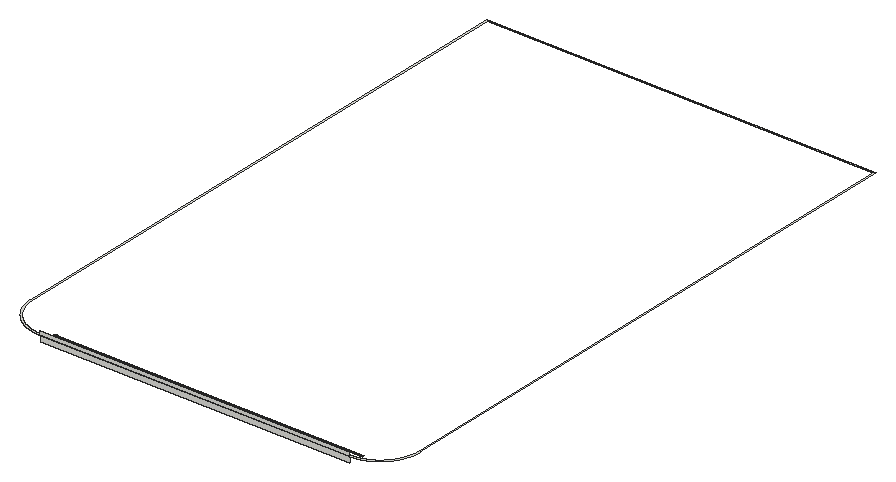
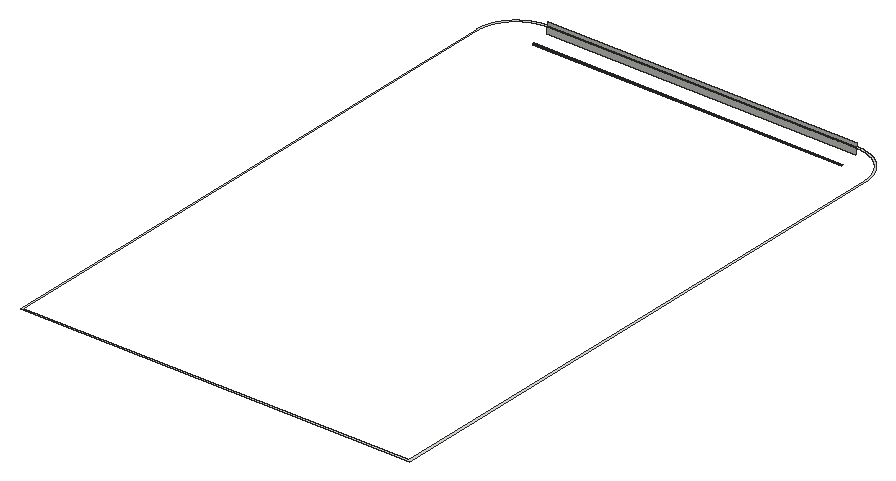
# SketchUp Ruby script. Lengths in inches.
U = 1.inch
M = Sketchup.active_model
def pt(a) = Geom::Point3d.new(a.map { |v| v * U })
def face(e, loops, mat)
  f = e.add_face(loops[0].map { |a| pt(a) })
  loops[1..].each { |l| e.add_face(l.map { |a| pt(a) }).erase! }
  f.material = f.back_material = mat if mat
  f
end
# faces: each face lists its corners as indices into pts; further lists are holes
def faces(e, pts, list, mat = nil) = list.each { |f| face(e, (f[0].is_a?(Array) ? f : [f]).map { |l| l.map { |i| pts[i] } }, mat) }
# xy, xz, yz: faces in a plane at the given z, y or x. An outline is a flat list of corners, or four numbers for a rectangle; further outlines are holes
def ring(l) = l.size == 4 ? [[l[0], l[1]], [l[2], l[1]], [l[2], l[3]], [l[0], l[3]]] : l.each_slice(2).to_a
def flat(e, list, mat, &to3) = list.each { |f| face(e, (f[0].is_a?(Array) ? f : [f]).map { |l| ring(l).map { |u, v| to3.(u, v) } }, mat) }
def xy(e, z, list, mat = nil) = flat(e, list, mat) { |x, y| [x, y, z] }
def xz(e, y, list, mat = nil) = flat(e, list, mat) { |x, z| [x, y, z] }
def yz(e, x, list, mat = nil) = flat(e, list, mat) { |y, z| [x, y, z] }
def lines(e, pts, list) = list.each { |a, b| e.add_line(pt(pts[a]), pt(pts[b])) }
# prism: a flat outline (further loops are holes) pulled along v
def prism(e, loops, v, mat = nil)
  f = face(e, loops, mat); d = Geom::Vector3d.new(v.map { |x| x * U })
  f.pushpull(f.normal.samedirection?(d) ? d.length : -d.length)
end
def box(e, o, s, mat = nil) = prism(e, [[o, [o[0] + s[0], o[1], o[2]], [o[0] + s[0], o[1] + s[1], o[2]], [o[0], o[1] + s[1], o[2]]]], [0, 0, s[2]], mat)
def at(x, y, z, deg = 0) = Geom::Transformation.translation(pt([x, y, z])) * Geom::Transformation.rotation(ORIGIN, Z_AXIS, deg.degrees)
def axes(o, x, y, z) = Geom::Transformation.new([*x, 0, *y, 0, *z, 0, *pt(o).to_a, 1])
def part(name) = M.definitions.add(name)
# library, detail: a bought-in or finely detailed component or shape, given as its bounding box
def library(name, o, s) = part(name).tap { |d| box(d.entities, o, s) }
def detail(e, o, s) = box(e.add_group.entities, o, s)
def put(e, d, t, mat = nil) = e.add_instance(d, t).tap { |i| i.material = mat if mat }
def group(e, t, mat = nil) = e.add_group.tap { |g| g.transformation = t; g.material = mat if mat }.entities
root = M.entities
xy(root,354.5,[[[38.61,204,38.21,204.01,37.82,204.02,37.43,204.04,37.04,204.0625,36.65,204.09,36.25,204.125,35.86,204.16,35.08,204.26,34.7,204.31,33.92,204.43,33.53,204.5,33.15,204.58,32.76,204.66,32.38,204.74,31.62,204.92,31.24,205.02,30.86,205.125,30.48,205.24,30.1,205.35,29.36,205.59,28.62,205.85,28.25,205.99,27.88,206.14,27.52,206.28,27.16,206.4375,26.8,206.59,26.44,206.76,26.08,206.92,25.73,207.09,25.03,207.45,24.69,207.64,24.34,207.83,24,208.02,23.66,208.22,23.33,208.42,22.99,208.63,22.66,208.84,22.33,209.06,22.01,209.28,21.6875,209.5,21.37,209.73,21.05,209.96,20.43,210.44,20.12,210.6875,19.82,210.93,19.52,211.1875,19.22,211.44,18.93,211.71,18.64,211.97,18.35,212.24,18.07,212.51,17.51,213.07,17.24,213.35,16.97,213.64,16.71,213.93,16.44,214.22,16.1875,214.52,15.93,214.82,15.6875,215.12,15.44,215.43,14.96,216.05,14.73,216.37,14.5,216.6875,14.28,217.01,14.06,217.33,13.84,217.66,13.63,217.99,13.42,218.33,13.22,218.66,13.02,219,12.83,219.34,12.64,219.69,12.45,220.03,12.09,220.73,11.92,221.08,11.76,221.44,11.59,221.8,11.4375,222.16,11.28,222.52,11.14,222.88,10.99,223.25,10.85,223.62,10.59,224.36,10.35,225.1,10.24,225.48,10.125,225.86,10.02,226.24,9.92,226.62,9.74,227.38,9.66,227.76,9.58,228.15,9.5,228.53,9.43,228.92,9.31,229.7,9.26,230.08,9.16,230.86,9.125,231.25,9.09,231.65,9.0625,232.04,9.04,232.43,9.02,232.82,9.01,233.21,9,233.61,9,660,300,660,300,233.61,299.99,233.21,299.98,232.82,299.96,232.43,299.9375,232.04,299.91,231.65,299.875,231.25,299.84,230.86,299.74,230.08,299.69,229.7,299.57,228.92,299.5,228.53,299.42,228.15,299.34,227.76,299.26,227.38,299.08,226.62,298.98,226.24,298.875,225.86,298.76,225.48,298.65,225.1,298.41,224.36,298.15,223.62,298.01,223.25,297.86,222.88,297.72,222.52,297.5625,222.16,297.41,221.8,297.24,221.44,297.08,221.08,296.91,220.73,296.55,220.03,296.36,219.69,296.17,219.34,295.98,219,295.78,218.66,295.58,218.33,295.37,217.99,295.16,217.66,294.94,217.33,294.72,217.01,294.5,216.6875,294.27,216.37,294.04,216.05,293.56,215.43,293.3125,215.12,293.07,214.82,292.8125,214.52,292.56,214.22,292.29,213.93,292.03,213.64,291.76,213.35,291.49,213.07,290.93,212.51,290.65,212.24,290.36,211.97,290.07,211.71,289.78,211.44,289.48,211.1875,289.18,210.93,288.88,210.6875,288.57,210.44,287.95,209.96,287.63,209.73,287.3125,209.5,286.99,209.28,286.67,209.06,286.34,208.84,286.01,208.63,285.67,208.42,285.34,208.22,285,208.02,284.66,207.83,284.31,207.64,283.97,207.45,283.27,207.09,282.92,206.92,282.56,206.76,282.2,206.59,281.84,206.4375,281.48,206.28,281.12,206.14,280.75,205.99,280.38,205.85,279.64,205.59,278.9,205.35,278.52,205.24,278.14,205.125,277.76,205.02,277.38,204.92,276.62,204.74,276.24,204.66,275.85,204.58,275.47,204.5,275.08,204.43,274.3,204.31,273.92,204.26,273.14,204.16,272.75,204.125,272.35,204.09,271.96,204.0625,271.57,204.04,271.18,204.02,270.79,204.01,270.39,204],[38.62,205,270.38,205,271.14,205.02,271.52,205.04,271.9,205.0625,272.28,205.09,272.65,205.12,273.41,205.2,273.79,205.25,274.16,205.3,274.54,205.36,274.91,205.42,275.28,205.49,275.66,205.56,276.03,205.63,276.4,205.72,276.77,205.8,277.14,205.89,277.51,205.99,277.87,206.09,278.24,206.19,278.6,206.3,279.68,206.66,280.04,206.79,280.39,206.93,280.75,207.06,281.8,207.51,282.14,207.66,282.48,207.83,282.83,207.99,283.17,208.16,283.5,208.34,283.84,208.51,284.83,209.08,285.15,209.27,285.47,209.47,286.43,210.1,287.05,210.54,287.35,210.76,287.65,210.99,287.95,211.23,288.25,211.46,288.54,211.7,289.12,212.2,289.4,212.45,289.69,212.7,289.96,212.96,290.24,213.23,290.51,213.49,290.77,213.76,291.04,214.04,291.3,214.31,291.55,214.6,291.8,214.88,292.3,215.46,292.54,215.75,292.77,216.05,293.01,216.35,293.24,216.65,293.46,216.95,293.9,217.57,294.53,218.53,294.73,218.85,294.92,219.17,295.49,220.16,295.66,220.5,295.84,220.83,296.01,221.17,296.17,221.52,296.34,221.86,296.49,222.2,296.94,223.25,297.07,223.61,297.21,223.96,297.34,224.32,297.7,225.4,297.81,225.76,297.91,226.13,298.01,226.49,298.11,226.86,298.2,227.23,298.28,227.6,298.37,227.97,298.44,228.34,298.51,228.72,298.58,229.09,298.64,229.46,298.7,229.84,298.75,230.21,298.8,230.59,298.88,231.35,298.91,231.72,298.9375,232.1,298.96,232.48,298.98,232.86,299,233.62,299,659,10,659,10,233.62,10.02,232.86,10.04,232.48,10.0625,232.1,10.09,231.72,10.12,231.35,10.2,230.59,10.25,230.21,10.3,229.84,10.36,229.46,10.42,229.09,10.49,228.72,10.56,228.34,10.63,227.97,10.72,227.6,10.8,227.23,10.89,226.86,10.99,226.49,11.09,226.13,11.19,225.76,11.3,225.4,11.66,224.32,11.79,223.96,11.93,223.61,12.06,223.25,12.51,222.2,12.66,221.86,12.83,221.52,12.99,221.17,13.16,220.83,13.34,220.5,13.51,220.16,14.08,219.17,14.27,218.85,14.47,218.53,15.1,217.57,15.54,216.95,15.76,216.65,15.99,216.35,16.23,216.05,16.46,215.75,16.7,215.46,17.2,214.88,17.45,214.6,17.7,214.31,17.96,214.04,18.23,213.76,18.49,213.49,18.76,213.23,19.04,212.96,19.31,212.7,19.6,212.45,19.88,212.2,20.46,211.7,20.75,211.46,21.05,211.23,21.35,210.99,21.65,210.76,21.95,210.54,22.57,210.1,23.53,209.47,23.85,209.27,24.17,209.08,25.16,208.51,25.5,208.34,25.83,208.16,26.17,207.99,26.52,207.83,26.86,207.66,27.2,207.51,28.25,207.06,28.61,206.93,28.96,206.79,29.32,206.66,30.4,206.3,30.76,206.19,31.13,206.09,31.49,205.99,31.86,205.89,32.23,205.8,32.6,205.72,32.97,205.63,33.34,205.56,33.72,205.49,34.09,205.42,34.46,205.36,34.84,205.3,35.21,205.25,35.59,205.2,36.35,205.12,36.72,205.09,37.1,205.0625,37.48,205.04,37.86,205.02]]])
xz(root,204,[[39,354.5,270,357]])
xz(root,205,[[39,349.5,270,354.5]])
xz(root,217,[[39,348,270,348.5]])
xz(root,218,[[39,348,270,348.5]])
